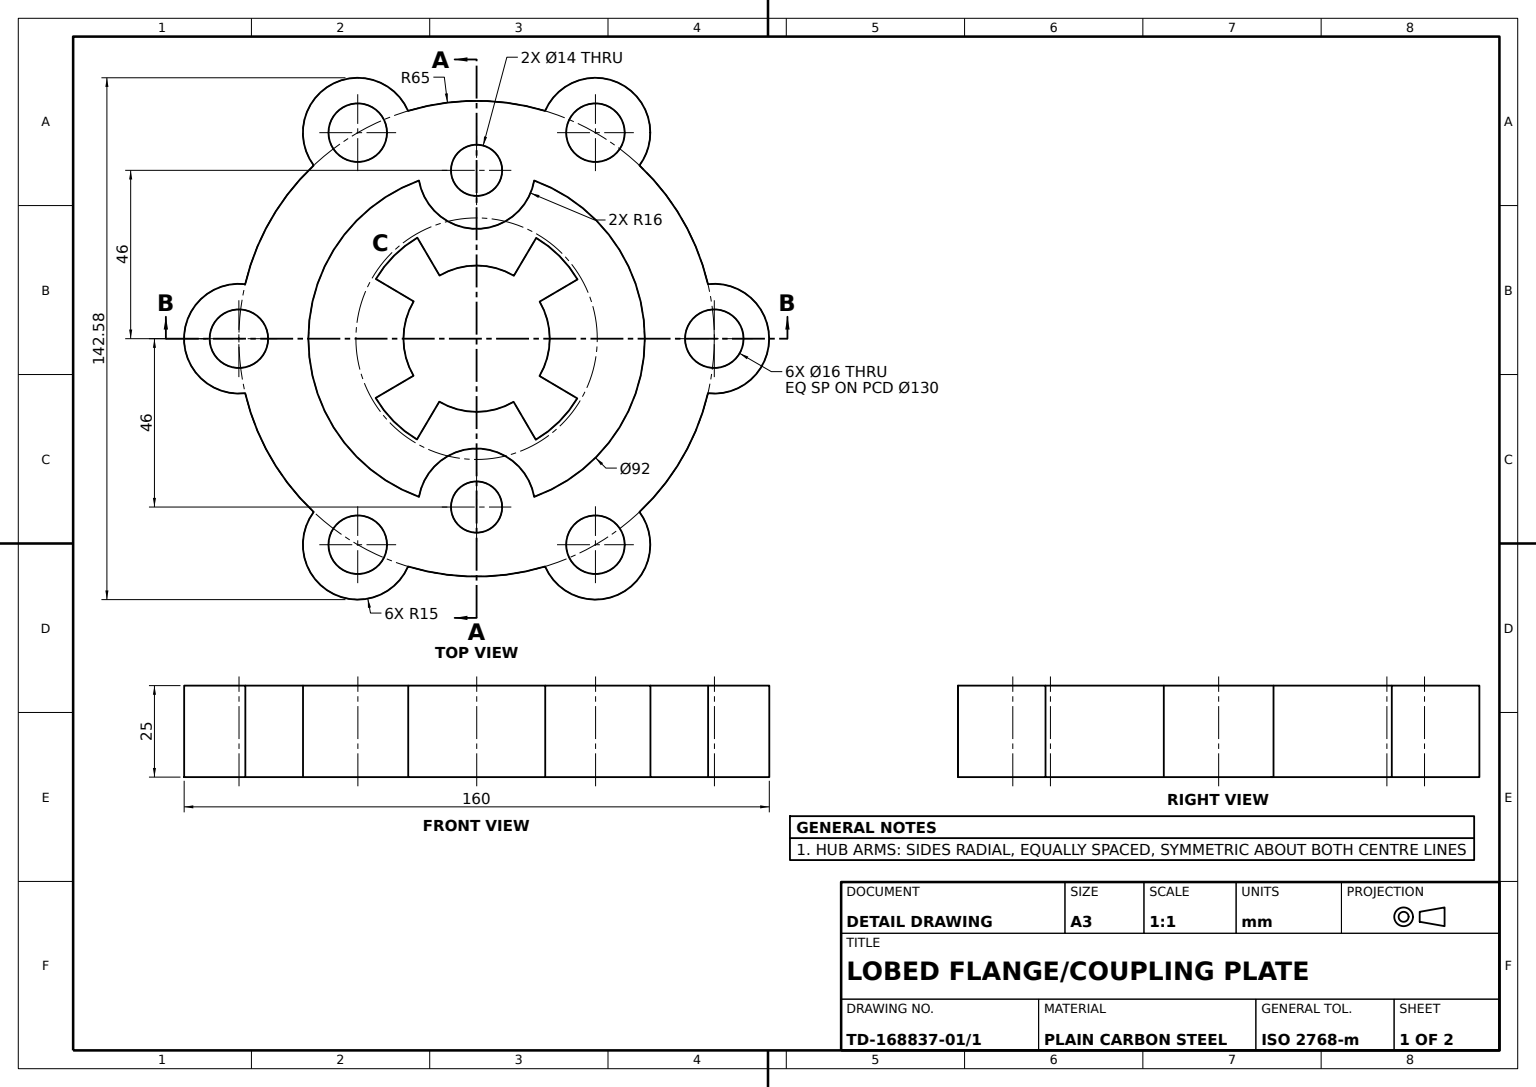
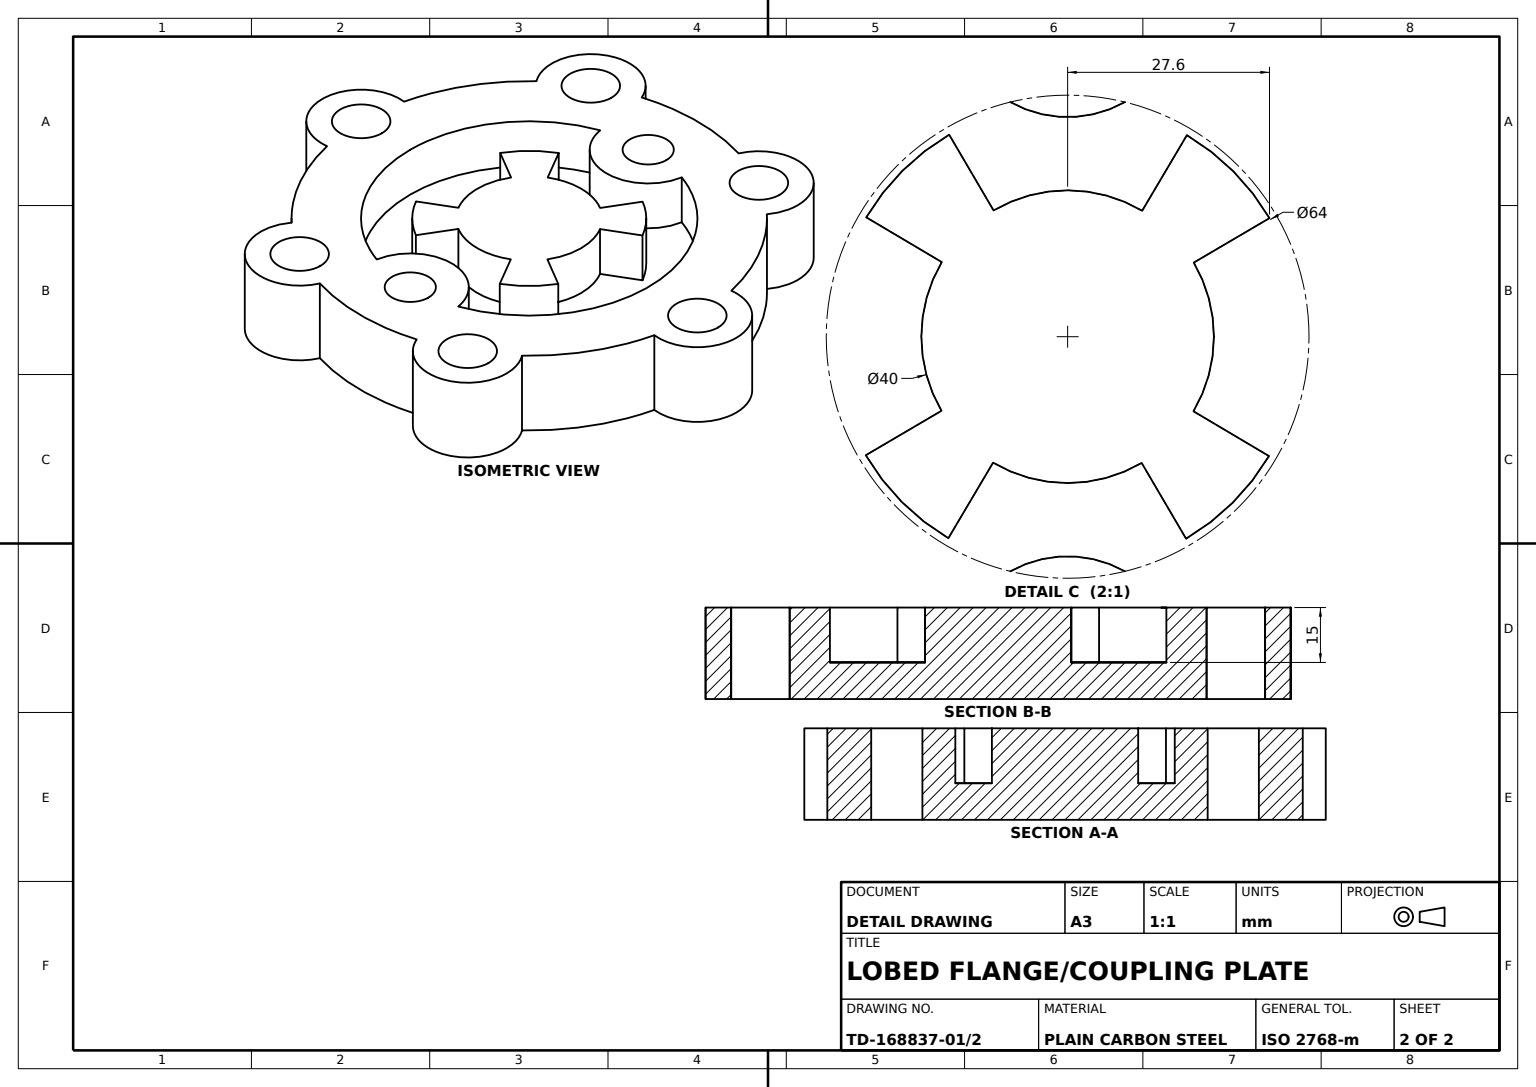
solid
v1 (-56.291651,25,-47.5)
v2 (-56.291651,0,-47.5)
e1 v1 v2 LINE
v3 (-62.242668,0,-18.730999)
e2 v2 v3 CIRCLE(AX(P(-56.291651,0,-32.5),D(0,1,0),D(0,0,1)),15)
v4 (-62.242668,25,-18.730999)
e3 v4 v3 LINE
e4 v1 v4 CIRCLE(AX(P(-56.291651,25,-32.5),D(0,1,0),D(0,0,1)),15)
face CYL(AX(P(-56.291651,25,-32.5),D(0,-1,0),D(0,0,-1)),15) [e1 e2 -e3 -e4]
v5 (43.217391,10,15.756176)
v6 (43.217391,10,-15.756176)
e5 v5 v6 CIRCLE(AX(P(46,10,0),D(0,-1,0),D(0,0,1)),16)
v7 (43.217391,25,15.756176)
e6 v5 v7 LINE
v8 (43.217391,25,-15.756176)
e7 v7 v8 CIRCLE(AX(P(46,25,0),D(0,-1,0),D(0,0,1)),16)
e8 v6 v8 LINE
face CYL(AX(P(46,10,0),D(0,1,0),D(0,0,1)),16) [-e5 e6 e7 -e8]
v9 (-43.217391,10,-15.756176)
v10 (-43.217391,25,-15.756176)
e9 v9 v10 LINE
e10 v6 v9 CIRCLE(AX(P(0,10,0),D(0,1,0),D(0,0,1)),46)
e11 v8 v10 CIRCLE(AX(P(0,25,0),D(0,1,0),D(0,0,1)),46)
face CYL(AX(P(0,10,0),D(0,1,0),D(0,0,1)),46) rev [-e9 -e10 e8 e11]
v11 (56.291651,0,24.5)
v12 (56.291651,0,40.5)
e12 v11 v12 CIRCLE(AX(P(56.291651,0,32.5),D(0,1,0),D(0,0,1)),8)
v13 (56.291651,25,24.5)
e13 v11 v13 LINE
v14 (56.291651,25,40.5)
e14 v13 v14 CIRCLE(AX(P(56.291651,25,32.5),D(0,1,0),D(0,0,1)),8)
e15 v12 v14 LINE
face CYL(AX(P(56.291651,0,32.5),D(0,1,0),D(0,0,1)),8) rev [-e12 e13 e14 -e15]
v15 (-43.217391,10,15.756176)
v16 (-43.217391,25,15.756176)
e16 v15 v16 LINE
v17 (0,25,46)
e17 v16 v17 CIRCLE(AX(P(0,25,0),D(0,1,0),D(0,0,1)),46)
v18 (0,10,46)
e18 v18 v17 LINE
e19 v15 v18 CIRCLE(AX(P(0,10,0),D(0,1,0),D(0,0,1)),46)
face CYL(AX(P(0,10,0),D(0,1,0),D(0,0,1)),46) rev [e16 e17 -e18 -e19]
v19 (-14.899813,25,-63.269231)
v20 (-14.899813,0,-63.269231)
e20 v19 v20 LINE
v21 (-47.342854,0,-44.538232)
e21 v20 v21 CIRCLE(AX(P(0,0,0),D(0,1,0),D(0,0,1)),65)
v22 (-47.342854,25,-44.538232)
e22 v22 v21 LINE
e23 v19 v22 CIRCLE(AX(P(0,25,0),D(0,1,0),D(0,0,1)),65)
face CYL(AX(P(0,25,0),D(0,-1,0),D(0,0,-1)),65) [e20 e21 -e22 -e23]
v23 (-14.899813,25,63.269231)
v24 (-14.899813,0,63.269231)
e24 v23 v24 LINE
v25 (-47.342854,25,44.538232)
e25 v25 v23 CIRCLE(AX(P(0,25,0),D(0,1,0),D(0,0,1)),65)
v26 (-47.342854,0,44.538232)
e26 v25 v26 LINE
e27 v26 v24 CIRCLE(AX(P(0,0,0),D(0,1,0),D(0,0,1)),65)
face CYL(AX(P(0,25,0),D(0,-1,0),D(0,0,-1)),65) [-e24 -e25 e26 e27]
v27 (-62.242668,25,18.730999)
e28 v27 v25 CIRCLE(AX(P(-56.291651,25,32.5),D(0,1,0),D(0,0,1)),15)
v28 (-62.242668,0,18.730999)
e29 v27 v28 LINE
e30 v28 v26 CIRCLE(AX(P(-56.291651,0,32.5),D(0,1,0),D(0,0,1)),15)
face CYL(AX(P(-56.291651,25,32.5),D(0,-1,0),D(0,0,-1)),15) [-e26 -e28 e29 e30]
v29 (-10.122628,25,-17.249127)
v30 (-16.196205,25,-27.598604)
e31 v29 v30 LINE
v31 (-10.122628,10,-17.249127)
e32 v29 v31 LINE
v32 (-16.196205,10,-27.598604)
e33 v31 v32 LINE
e34 v30 v32 LINE
face PLANE(AX(P(-10.122628,25,-17.249127),D(-0.862456369,0,0.506131417),D(0.506131417,0,0.862456369))) rev [-e31 e32 e33 -e34]
e35 v9 v15 CIRCLE(AX(P(-46,10,0),D(0,-1,0),D(0,0,1)),16)
e36 v18 v5 CIRCLE(AX(P(0,10,0),D(0,1,0),D(0,0,1)),46)
v33 (-27.532796,10,-16.307824)
e37 v32 v33 CIRCLE(AX(P(0,10,0),D(0,1,0),D(0,0,1)),32)
v34 (0,10,-20)
e38 v34 v31 CIRCLE(AX(P(0,10,0),D(0,1,0),D(0,0,1)),20)
v35 (10.19239,10,-17.207998)
e39 v35 v34 CIRCLE(AX(P(0,10,0),D(0,1,0),D(0,0,1)),20)
v36 (16.307824,10,-27.532796)
e40 v36 v35 LINE
v37 (27.598604,10,-16.196205)
e41 v37 v36 CIRCLE(AX(P(0,10,0),D(0,1,0),D(0,0,1)),32)
v38 (17.249127,10,-10.122628)
e42 v38 v37 LINE
v39 (17.207998,10,10.19239)
e43 v39 v38 CIRCLE(AX(P(0,10,0),D(0,1,0),D(0,0,1)),20)
v40 (27.532796,10,16.307824)
e44 v40 v39 LINE
v41 (16.196205,10,27.598604)
e45 v41 v40 CIRCLE(AX(P(0,10,0),D(0,1,0),D(0,0,1)),32)
v42 (10.122628,10,17.249127)
e46 v42 v41 LINE
v43 (-10.19239,10,17.207998)
e47 v43 v42 CIRCLE(AX(P(0,10,0),D(0,1,0),D(0,0,1)),20)
v44 (-16.307824,10,27.532796)
e48 v44 v43 LINE
v45 (-27.598604,10,16.196205)
e49 v45 v44 CIRCLE(AX(P(0,10,0),D(0,1,0),D(0,0,1)),32)
v46 (-17.249127,10,10.122628)
e50 v46 v45 LINE
v47 (-17.207998,10,-10.19239)
e51 v47 v46 CIRCLE(AX(P(0,10,0),D(0,1,0),D(0,0,1)),20)
e52 v33 v47 LINE
face PLANE(AX(P(23,10,0),D(0,1,0),D(0,0,1))) [e35 e19 e36 e5 e10] [-e37 -e33 -e38 -e39 -e40 -e41 -e42 -e43 -e44 -e45 -e46 -e47 -e48 -e49 -e50 -e51 -e52]
v48 (-56.291651,0,-24.5)
v49 (-56.291651,25,-24.5)
e53 v48 v49 LINE
v50 (-56.291651,0,-40.5)
e54 v50 v48 CIRCLE(AX(P(-56.291651,0,-32.5),D(0,1,0),D(0,0,1)),8)
v51 (-56.291651,25,-40.5)
e55 v50 v51 LINE
e56 v51 v49 CIRCLE(AX(P(-56.291651,25,-32.5),D(0,1,0),D(0,0,1)),8)
face CYL(AX(P(-56.291651,0,-32.5),D(0,1,0),D(0,0,1)),8) rev [-e53 -e54 e55 e56]
e57 v48 v50 CIRCLE(AX(P(-56.291651,0,-32.5),D(0,1,0),D(0,0,1)),8)
e58 v49 v51 CIRCLE(AX(P(-56.291651,25,-32.5),D(0,1,0),D(0,0,1)),8)
face CYL(AX(P(-56.291651,0,-32.5),D(0,1,0),D(0,0,1)),8) rev [-e55 -e57 e53 e58]
v52 (-17.207998,25,-10.19239)
e59 v52 v47 LINE
v53 (-17.249127,25,10.122628)
e60 v53 v46 LINE
e61 v52 v53 CIRCLE(AX(P(0,25,0),D(0,1,0),D(0,0,1)),20)
face CYL(AX(P(0,25,0),D(0,-1,0),D(0,0,-1)),20) [e59 e51 -e60 -e61]
v54 (-27.598604,25,16.196205)
e62 v53 v54 LINE
v55 (-16.307824,25,27.532796)
e63 v54 v55 CIRCLE(AX(P(0,25,0),D(0,1,0),D(0,0,1)),32)
v56 (-10.19239,25,17.207998)
e64 v55 v56 LINE
v57 (10.122628,25,17.249127)
e65 v56 v57 CIRCLE(AX(P(0,25,0),D(0,1,0),D(0,0,1)),20)
v58 (16.196205,25,27.598604)
e66 v57 v58 LINE
v59 (27.532796,25,16.307824)
e67 v58 v59 CIRCLE(AX(P(0,25,0),D(0,1,0),D(0,0,1)),32)
v60 (17.207998,25,10.19239)
e68 v59 v60 LINE
v61 (17.249127,25,-10.122628)
e69 v60 v61 CIRCLE(AX(P(0,25,0),D(0,1,0),D(0,0,1)),20)
v62 (27.598604,25,-16.196205)
e70 v61 v62 LINE
v63 (16.307824,25,-27.532796)
e71 v62 v63 CIRCLE(AX(P(0,25,0),D(0,1,0),D(0,0,1)),32)
v64 (10.19239,25,-17.207998)
e72 v63 v64 LINE
v65 (0,25,-20)
e73 v64 v65 CIRCLE(AX(P(0,25,0),D(0,1,0),D(0,0,1)),20)
e74 v65 v29 CIRCLE(AX(P(0,25,0),D(0,1,0),D(0,0,1)),20)
v66 (-27.532796,25,-16.307824)
e75 v30 v66 CIRCLE(AX(P(0,25,0),D(0,1,0),D(0,0,1)),32)
e76 v66 v52 LINE
face PLANE(AX(P(0,25,0),D(0,1,0),D(0,0,1))) [e62 e63 e64 e65 e66 e67 e68 e69 e70 e71 e72 e73 e74 e31 e75 e76 e61]
v67 (14.899813,0,63.269231)
e77 v24 v67 CIRCLE(AX(P(0,0,65),D(0,1,0),D(0,0,1)),15)
v68 (14.899813,25,63.269231)
e78 v68 v67 LINE
e79 v23 v68 CIRCLE(AX(P(0,25,65),D(0,1,0),D(0,0,1)),15)
face CYL(AX(P(0,25,65),D(0,-1,0),D(0,0,-1)),15) [e24 e77 -e78 -e79]
e80 v64 v35 LINE
e81 v63 v36 LINE
face PLANE(AX(P(10.19239,25,-17.207998),D(0.860399884,0,0.509619504),D(0.509619504,0,-0.860399884))) rev [-e80 -e72 e81 e40]
v69 (14.899813,25,-63.269231)
v70 (14.899813,0,-63.269231)
e82 v69 v70 LINE
v71 (47.342854,25,-44.538232)
e83 v71 v69 CIRCLE(AX(P(0,25,0),D(0,1,0),D(0,0,1)),65)
v72 (47.342854,0,-44.538232)
e84 v71 v72 LINE
e85 v72 v70 CIRCLE(AX(P(0,0,0),D(0,1,0),D(0,0,1)),65)
face CYL(AX(P(0,25,0),D(0,-1,0),D(0,0,-1)),65) [-e82 -e83 e84 e85]
e86 v62 v37 LINE
face CYL(AX(P(0,25,0),D(0,-1,0),D(0,0,-1)),32) [-e81 -e71 e86 e41]
e87 v12 v11 CIRCLE(AX(P(56.291651,0,32.5),D(0,1,0),D(0,0,1)),8)
e88 v14 v13 CIRCLE(AX(P(56.291651,25,32.5),D(0,1,0),D(0,0,1)),8)
face CYL(AX(P(56.291651,0,32.5),D(0,1,0),D(0,0,1)),8) rev [-e87 e15 e88 -e13]
e89 v65 v34 LINE
face CYL(AX(P(0,25,0),D(0,-1,0),D(0,0,-1)),20) [e89 e38 -e32 -e74]
e90 v54 v45 LINE
face PLANE(AX(P(-17.249127,25,10.122628),D(0.506131417,0,0.862456369),D(0.862456369,0,-0.506131417))) rev [-e62 e60 e50 -e90]
e91 v4 v27 CIRCLE(AX(P(0,25,0),D(0,1,0),D(0,0,1)),65)
e92 v3 v28 CIRCLE(AX(P(0,0,0),D(0,1,0),D(0,0,1)),65)
face CYL(AX(P(0,25,0),D(0,-1,0),D(0,0,-1)),65) [-e91 e3 e92 -e29]
v73 (-46,25,-7)
v74 (-46,25,7)
e93 v73 v74 CIRCLE(AX(P(-46,25,0),D(0,1,0),D(0,0,1)),7)
e94 v74 v73 CIRCLE(AX(P(-46,25,0),D(0,1,0),D(0,0,1)),7)
e95 v17 v7 CIRCLE(AX(P(0,25,0),D(0,1,0),D(0,0,1)),46)
e96 v10 v16 CIRCLE(AX(P(-46,25,0),D(0,-1,0),D(0,0,1)),16)
v75 (0,25,-57)
v76 (0,25,-73)
e97 v75 v76 CIRCLE(AX(P(0,25,-65),D(0,1,0),D(0,0,1)),8)
e98 v76 v75 CIRCLE(AX(P(0,25,-65),D(0,1,0),D(0,0,1)),8)
v77 (46,25,7)
v78 (46,25,-7)
e99 v77 v78 CIRCLE(AX(P(46,25,0),D(0,1,0),D(0,0,1)),7)
e100 v78 v77 CIRCLE(AX(P(46,25,0),D(0,1,0),D(0,0,1)),7)
v79 (56.291651,25,-40.5)
v80 (56.291651,25,-24.5)
e101 v79 v80 CIRCLE(AX(P(56.291651,25,-32.5),D(0,1,0),D(0,0,1)),8)
e102 v80 v79 CIRCLE(AX(P(56.291651,25,-32.5),D(0,1,0),D(0,0,1)),8)
v81 (47.342854,25,44.538232)
e103 v68 v81 CIRCLE(AX(P(0,25,0),D(0,1,0),D(0,0,1)),65)
v82 (62.242668,25,18.730999)
e104 v81 v82 CIRCLE(AX(P(56.291651,25,32.5),D(0,1,0),D(0,0,1)),15)
v83 (62.242668,25,-18.730999)
e105 v82 v83 CIRCLE(AX(P(0,25,0),D(0,1,0),D(0,0,1)),65)
v84 (56.291651,25,-47.5)
e106 v83 v84 CIRCLE(AX(P(56.291651,25,-32.5),D(0,1,0),D(0,0,1)),15)
e107 v84 v71 CIRCLE(AX(P(56.291651,25,-32.5),D(0,1,0),D(0,0,1)),15)
v85 (0,25,-80)
e108 v69 v85 CIRCLE(AX(P(0,25,-65),D(0,1,0),D(0,0,1)),15)
e109 v85 v19 CIRCLE(AX(P(0,25,-65),D(0,1,0),D(0,0,1)),15)
e110 v22 v1 CIRCLE(AX(P(-56.291651,25,-32.5),D(0,1,0),D(0,0,1)),15)
v86 (0,25,73)
v87 (0,25,57)
e111 v86 v87 CIRCLE(AX(P(0,25,65),D(0,1,0),D(0,0,1)),8)
e112 v87 v86 CIRCLE(AX(P(0,25,65),D(0,1,0),D(0,0,1)),8)
v88 (-56.291651,25,24.5)
v89 (-56.291651,25,40.5)
e113 v88 v89 CIRCLE(AX(P(-56.291651,25,32.5),D(0,1,0),D(0,0,1)),8)
e114 v89 v88 CIRCLE(AX(P(-56.291651,25,32.5),D(0,1,0),D(0,0,1)),8)
face PLANE(AX(P(28.145826,25,-16.25),D(0,1,0),D(0,0,1))) [-e93 -e94] [-e7 -e95 -e17 -e96 -e11] [-e97 -e98] [-e99 -e100] [-e56 -e58] [-e101 -e102] [e25 e79 e103 e104 e105 e106 e107 e83 e108 e109 e23 e110 e4 e91 e28] [-e88 -e14] [-e111 -e112] [-e113 -e114]
e115 v61 v38 LINE
face PLANE(AX(P(17.249127,25,-10.122628),D(-0.506131417,0,-0.862456369),D(-0.862456369,0,0.506131417))) rev [e115 e42 -e86 -e70]
v90 (-46,0,7)
v91 (-46,0,-7)
e116 v90 v91 CIRCLE(AX(P(-46,0,0),D(0,1,0),D(0,0,1)),7)
e117 v90 v74 LINE
e118 v91 v73 LINE
face CYL(AX(P(-46,0,0),D(0,1,0),D(0,0,1)),7) rev [-e116 e117 e94 -e118]
v92 (56.291651,0,-47.5)
e119 v84 v92 LINE
e120 v92 v72 CIRCLE(AX(P(56.291651,0,-32.5),D(0,1,0),D(0,0,1)),15)
face CYL(AX(P(56.291651,25,-32.5),D(0,-1,0),D(0,0,-1)),15) [-e84 -e107 e119 e120]
e121 v59 v40 LINE
e122 v60 v39 LINE
face PLANE(AX(P(17.207998,25,10.19239),D(-0.509619504,0,0.860399884),D(0.860399884,0,0.509619504))) rev [-e68 e121 e44 -e122]
v93 (-56.291651,0,24.5)
v94 (-56.291651,0,40.5)
e123 v93 v94 CIRCLE(AX(P(-56.291651,0,32.5),D(0,1,0),D(0,0,1)),8)
e124 v93 v88 LINE
e125 v94 v89 LINE
face CYL(AX(P(-56.291651,0,32.5),D(0,1,0),D(0,0,1)),8) rev [-e123 e124 e113 -e125]
e126 v66 v33 LINE
face CYL(AX(P(0,25,0),D(0,-1,0),D(0,0,-1)),32) [-e75 e34 e37 -e126]
face CYL(AX(P(0,25,0),D(0,-1,0),D(0,0,-1)),20) [e43 -e115 -e69 e122]
v95 (62.242668,0,18.730999)
v96 (62.242668,0,-18.730999)
e127 v95 v96 CIRCLE(AX(P(0,0,0),D(0,1,0),D(0,0,1)),65)
e128 v83 v96 LINE
e129 v82 v95 LINE
face CYL(AX(P(0,25,0),D(0,-1,0),D(0,0,-1)),65) [e127 -e128 -e105 e129]
v97 (0,0,-80)
e130 v70 v97 CIRCLE(AX(P(0,0,-65),D(0,1,0),D(0,0,1)),15)
e131 v85 v97 LINE
face CYL(AX(P(0,25,-65),D(0,-1,0),D(0,0,-1)),15) [e82 e130 -e131 -e108]
e132 v91 v90 CIRCLE(AX(P(-46,0,0),D(0,1,0),D(0,0,1)),7)
face CYL(AX(P(-46,0,0),D(0,1,0),D(0,0,1)),7) rev [-e132 e118 e93 -e117]
e133 v58 v41 LINE
e134 v57 v42 LINE
face PLANE(AX(P(10.122628,25,17.249127),D(0.862456369,0,-0.506131417),D(-0.506131417,0,-0.862456369))) rev [e46 -e133 -e66 e134]
face CYL(AX(P(0,10,0),D(0,1,0),D(0,0,1)),46) rev [-e36 e18 e95 -e6]
v98 (0,0,-73)
e135 v98 v76 LINE
v99 (0,0,-57)
e136 v99 v98 CIRCLE(AX(P(0,0,-65),D(0,1,0),D(0,0,1)),8)
e137 v99 v75 LINE
face CYL(AX(P(0,0,-65),D(0,1,0),D(0,0,1)),8) rev [e97 -e135 -e136 e137]
face CYL(AX(P(-46,10,0),D(0,1,0),D(0,0,1)),16) [e96 -e16 -e35 e9]
v100 (56.291651,0,-40.5)
v101 (56.291651,0,-24.5)
e138 v100 v101 CIRCLE(AX(P(56.291651,0,-32.5),D(0,1,0),D(0,0,1)),8)
e139 v101 v100 CIRCLE(AX(P(56.291651,0,-32.5),D(0,1,0),D(0,0,1)),8)
e140 v94 v93 CIRCLE(AX(P(-56.291651,0,32.5),D(0,1,0),D(0,0,1)),8)
v102 (46,0,7)
v103 (46,0,-7)
e141 v102 v103 CIRCLE(AX(P(46,0,0),D(0,1,0),D(0,0,1)),7)
e142 v103 v102 CIRCLE(AX(P(46,0,0),D(0,1,0),D(0,0,1)),7)
e143 v98 v99 CIRCLE(AX(P(0,0,-65),D(0,1,0),D(0,0,1)),8)
v104 (0,0,57)
v105 (0,0,73)
e144 v104 v105 CIRCLE(AX(P(0,0,65),D(0,1,0),D(0,0,1)),8)
e145 v105 v104 CIRCLE(AX(P(0,0,65),D(0,1,0),D(0,0,1)),8)
e146 v21 v2 CIRCLE(AX(P(-56.291651,0,-32.5),D(0,1,0),D(0,0,1)),15)
e147 v97 v20 CIRCLE(AX(P(0,0,-65),D(0,1,0),D(0,0,1)),15)
e148 v96 v92 CIRCLE(AX(P(56.291651,0,-32.5),D(0,1,0),D(0,0,1)),15)
v106 (47.342854,0,44.538232)
e149 v106 v95 CIRCLE(AX(P(56.291651,0,32.5),D(0,1,0),D(0,0,1)),15)
e150 v67 v106 CIRCLE(AX(P(0,0,0),D(0,1,0),D(0,0,1)),65)
face PLANE(AX(P(28.145826,0,-16.25),D(0,1,0),D(0,0,1))) rev [e12 e87] [e138 e139] [e123 e140] [e141 e142] [e143 e136] [e57 e54] [e144 e145] [e116 e132] [-e77 -e27 -e30 -e92 -e2 -e146 -e21 -e147 -e130 -e85 -e120 -e148 -e127 -e149 -e150]
e151 v104 v87 LINE
e152 v105 v86 LINE
face CYL(AX(P(0,0,65),D(0,1,0),D(0,0,1)),8) rev [-e144 e151 e112 -e152]
face CYL(AX(P(-56.291651,0,32.5),D(0,1,0),D(0,0,1)),8) rev [e125 e114 -e124 -e140]
e153 v81 v106 LINE
face CYL(AX(P(56.291651,25,32.5),D(0,-1,0),D(0,0,-1)),15) [-e104 e153 e149 -e129]
e154 v102 v77 LINE
e155 v103 v78 LINE
face CYL(AX(P(46,0,0),D(0,1,0),D(0,0,1)),7) rev [-e154 -e142 e155 e100]
face CYL(AX(P(56.291651,25,-32.5),D(0,-1,0),D(0,0,-1)),15) [e148 -e119 -e106 e128]
face CYL(AX(P(46,0,0),D(0,1,0),D(0,0,1)),7) rev [-e155 -e141 e154 e99]
e156 v56 v43 LINE
face CYL(AX(P(0,25,0),D(0,-1,0),D(0,0,-1)),20) [e47 -e134 -e65 e156]
face CYL(AX(P(0,25,-65),D(0,-1,0),D(0,0,-1)),15) [e147 -e20 -e109 e131]
face CYL(AX(P(0,0,-65),D(0,1,0),D(0,0,1)),8) rev [-e143 e135 e98 -e137]
e157 v55 v44 LINE
face PLANE(AX(P(-10.19239,25,17.207998),D(-0.860399884,0,-0.509619504),D(-0.509619504,0,0.860399884))) rev [e48 -e156 -e64 e157]
face CYL(AX(P(0,0,65),D(0,1,0),D(0,0,1)),8) rev [e152 e111 -e151 -e145]
face CYL(AX(P(0,25,0),D(0,-1,0),D(0,0,-1)),32) [-e157 -e63 e90 e49]
face CYL(AX(P(0,25,0),D(0,-1,0),D(0,0,-1)),20) [e80 e39 -e89 -e73]
face PLANE(AX(P(-17.207998,25,-10.19239),D(0.509619504,0,-0.860399884),D(-0.860399884,0,-0.509619504))) rev [-e76 e126 e52 -e59]
e158 v101 v80 LINE
e159 v100 v79 LINE
face CYL(AX(P(56.291651,0,-32.5),D(0,1,0),D(0,0,1)),8) rev [-e139 e158 e102 -e159]
face CYL(AX(P(0,25,0),D(0,-1,0),D(0,0,-1)),32) [-e121 -e67 e133 e45]
face CYL(AX(P(-56.291651,25,-32.5),D(0,-1,0),D(0,0,-1)),15) [e146 -e1 -e110 e22]
face CYL(AX(P(56.291651,0,-32.5),D(0,1,0),D(0,0,1)),8) rev [e159 e101 -e158 -e138]
face CYL(AX(P(0,25,0),D(0,-1,0),D(0,0,-1)),65) [-e153 -e103 e78 e150]
